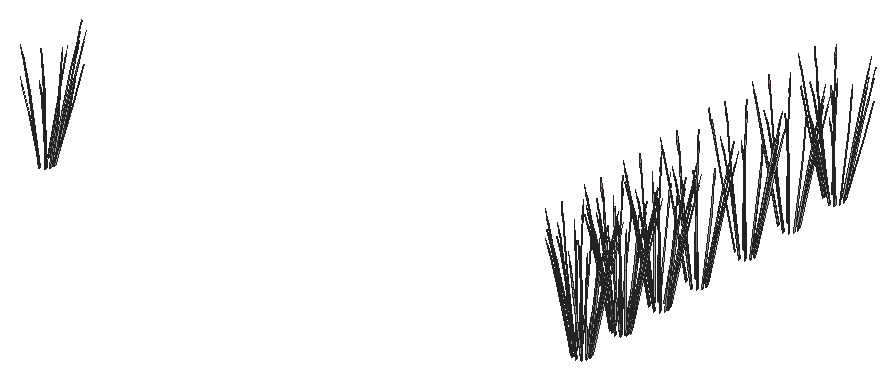
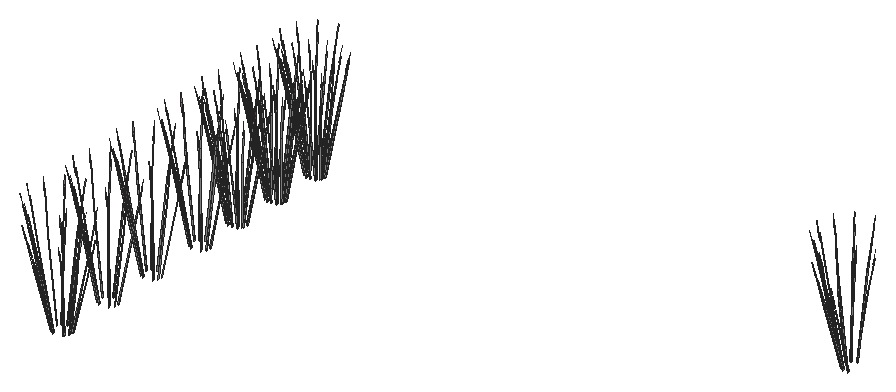
# SketchUp Ruby script. Lengths in inches.
U = 1.inch
M = Sketchup.active_model
def pt(a) = Geom::Point3d.new(a.map { |v| v * U })
def face(e, loops, mat)
  f = e.add_face(loops[0].map { |a| pt(a) })
  loops[1..].each { |l| e.add_face(l.map { |a| pt(a) }).erase! }
  f.material = f.back_material = mat if mat
  f
end
# faces: each face lists its corners as indices into pts; further lists are holes
def faces(e, pts, list, mat = nil) = list.each { |f| face(e, (f[0].is_a?(Array) ? f : [f]).map { |l| l.map { |i| pts[i] } }, mat) }
# xy, xz, yz: faces in a plane at the given z, y or x. An outline is a flat list of corners, or four numbers for a rectangle; further outlines are holes
def ring(l) = l.size == 4 ? [[l[0], l[1]], [l[2], l[1]], [l[2], l[3]], [l[0], l[3]]] : l.each_slice(2).to_a
def flat(e, list, mat, &to3) = list.each { |f| face(e, (f[0].is_a?(Array) ? f : [f]).map { |l| ring(l).map { |u, v| to3.(u, v) } }, mat) }
def xy(e, z, list, mat = nil) = flat(e, list, mat) { |x, y| [x, y, z] }
def xz(e, y, list, mat = nil) = flat(e, list, mat) { |x, z| [x, y, z] }
def yz(e, x, list, mat = nil) = flat(e, list, mat) { |y, z| [x, y, z] }
def lines(e, pts, list) = list.each { |a, b| e.add_line(pt(pts[a]), pt(pts[b])) }
# prism: a flat outline (further loops are holes) pulled along v
def prism(e, loops, v, mat = nil)
  f = face(e, loops, mat); d = Geom::Vector3d.new(v.map { |x| x * U })
  f.pushpull(f.normal.samedirection?(d) ? d.length : -d.length)
end
def box(e, o, s, mat = nil) = prism(e, [[o, [o[0] + s[0], o[1], o[2]], [o[0] + s[0], o[1] + s[1], o[2]], [o[0], o[1] + s[1], o[2]]]], [0, 0, s[2]], mat)
def at(x, y, z, deg = 0) = Geom::Transformation.translation(pt([x, y, z])) * Geom::Transformation.rotation(ORIGIN, Z_AXIS, deg.degrees)
def axes(o, x, y, z) = Geom::Transformation.new([*x, 0, *y, 0, *z, 0, *pt(o).to_a, 1])
def part(name) = M.definitions.add(name)
# library, detail: a bought-in or finely detailed component or shape, given as its bounding box
def library(name, o, s) = part(name).tap { |d| box(d.entities, o, s) }
def detail(e, o, s) = box(e.add_group.entities, o, s)
def put(e, d, t, mat = nil) = e.add_instance(d, t).tap { |i| i.material = mat if mat }
def group(e, t, mat = nil) = e.add_group.tap { |g| g.transformation = t; g.material = mat if mat }.entities
root = M.entities
M.materials.add("LightPink_Translucent").color = [144, 107, 117]
M.materials["LightPink_Translucent"].alpha = 0.75
M.materials.add("[_0053_Ivory_]").color = [200, 200, 200]
c1 = part("blade")
p = [[2.15,0.21,22],[0,0.17,0],[0.09,0.45,0],[2.18,0.31,22],[2.29,0.31,22],[0.38,0.45,0],
  [2.48,0.24,33],[2.49,0.24,33],[2.48,0.22,33]]
faces(c1.entities,p,[[0,1,2,3],[4,5,2,3],[6,3,4,7],[8,0,3,6]])
c2 = part("seeds")
p = [[0.3,-0.1,1.38],[-0.01,-0.03,1.59],[-0.01,-0.03,0.03],[0.14,-0.07,-0.07],[0.29,-0.03,3],[0.15,0.01,3.11]]
faces(c2.entities,p,[[0,1,2,3],[1,0,4,5]],"LightPink_Translucent")
c3 = part("blade with seeds")
put(c3.entities,c1,at(0,0,0))
put(c3.entities,c2,axes([2.4,0.25,30.99],[1.5799,-0.05474,1.17369],[-0.12525,1.92788,0.29478],[-0.07173,-0.02425,1.56792]))
put(root,c3,axes([483.9375,105.12,131.38],[-0.44753,0.21372,0.0643],[-0.21905,-0.38973,0.50621],[0.04322,0.1718,0.77189]),"[_0053_Ivory_]")
put(root,c3,axes([485.24,99.58,131.38],[0.44753,-0.21372,0.0643],[0.21905,0.38973,0.50621],[-0.04322,-0.1718,0.77189]),"[_0053_Ivory_]")
put(root,c3,axes([485.08,99.62,131.39],[0.59846,0.1644,0.48003],[-0.20464,0.54049,0.3958],[-0.03596,-0.21255,0.9933]),"[_0053_Ivory_]")
put(root,c3,axes([485.59,104.95,131.39],[-0.60408,0.14432,0.48003],[-0.10484,-0.56611,0.3958],[0.14207,0.16684,0.9933]),"[_0053_Ivory_]")
put(root,c3,axes([485.47,105.06,131.38],[-0.27604,0.39948,0.0643],[-0.39309,-0.23258,0.50621],[0.12709,0.12808,0.77189]),"[_0053_Ivory_]")
put(root,c3,axes([486.6,100.26,131.38],[0.49911,0.0293,0.0643],[-0.01368,0.44245,0.50621],[0.05223,-0.16948,0.77189]),"[_0053_Ivory_]")
put(root,c3,axes([486.44,100.22,131.39],[0.43249,0.42907,0.48003],[-0.45929,0.37004,0.3958],[0.07978,-0.2013,0.9933]),"[_0053_Ivory_]")
put(root,c3,axes([486.77,104.27,131.38],[-0.03058,0.47819,0.0643],[-0.4618,-0.01311,0.50621],[0.1769,0.05004,0.77189]),"[_0053_Ivory_]")
put(root,c3,axes([486.8125,104.12,131.39],[-0.44783,0.41436,0.48003],[-0.38623,-0.44004,0.3958],[0.21011,0.07643,0.9933]),"[_0053_Ivory_]")
put(root,c3,axes([487.42,101.5,131.38],[0.41695,0.26447,0.0643],[-0.24275,0.37662,0.50621],[0.13368,-0.12176,0.77189]),"[_0053_Ivory_]")
put(root,c3,axes([487.3,101.39,131.39],[0.15063,0.57876,0.48003],[-0.59087,0.10045,0.3958],[0.17414,-0.13612,0.9933]),"[_0053_Ivory_]")
put(root,c3,axes([487.48,102.97,131.38],[0.22307,0.42878,0.0643],[-0.40677,0.20987,0.50621],[0.17931,-0.04141,0.77189]),"[_0053_Ivory_]")
put(root,c3,axes([487.4375,102.82,131.39],[-0.17159,0.57338,0.48003],[-0.56413,-0.19607,0.3958],[0.22185,-0.03446,0.9933]),"[_0053_Ivory_]")
put(root,c3,axes([640.98,108.99,131.39],[0.17159,-0.57338,0.48003],[0.56413,0.19607,0.3958],[-0.22185,0.03446,0.9933]),"[_0053_Ivory_]")
put(root,c3,axes([640.98,124.05,131.39],[0.17159,-0.57338,0.48003],[0.56413,0.19607,0.3958],[-0.22185,0.03446,0.9933]),"[_0053_Ivory_]")
put(root,c3,axes([640.98,138.97,131.39],[0.17159,-0.57338,0.48003],[0.56413,0.19607,0.3958],[-0.22185,0.03446,0.9933]),"[_0053_Ivory_]")
put(root,c3,axes([640.98,153.24,131.39],[0.17159,-0.57338,0.48003],[0.56413,0.19607,0.3958],[-0.22185,0.03446,0.9933]),"[_0053_Ivory_]")
put(root,c3,axes([640.98,171.73,131.39],[0.17159,-0.57338,0.48003],[0.56413,0.19607,0.3958],[-0.22185,0.03446,0.9933]),"[_0053_Ivory_]")
put(root,c3,axes([640.98,188.49,131.39],[0.17159,-0.57338,0.48003],[0.56413,0.19607,0.3958],[-0.22185,0.03446,0.9933]),"[_0053_Ivory_]")
put(root,c3,axes([640.98,206.08,131.39],[0.17159,-0.57338,0.48003],[0.56413,0.19607,0.3958],[-0.22185,0.03446,0.9933]),"[_0053_Ivory_]")
put(root,c3,axes([640.93,205.93,131.38],[-0.22307,-0.42878,0.0643],[0.40677,-0.20987,0.50621],[-0.17931,0.04141,0.77189]),"[_0053_Ivory_]")
put(root,c3,axes([641.11,110.42,131.39],[-0.15063,-0.57876,0.48003],[0.59087,-0.10045,0.3958],[-0.17414,0.13612,0.9933]),"[_0053_Ivory_]")
put(root,c3,axes([641.11,125.48,131.39],[-0.15063,-0.57876,0.48003],[0.59087,-0.10045,0.3958],[-0.17414,0.13612,0.9933]),"[_0053_Ivory_]")
put(root,c3,axes([641.11,140.4,131.39],[-0.15063,-0.57876,0.48003],[0.59087,-0.10045,0.3958],[-0.17414,0.13612,0.9933]),"[_0053_Ivory_]")
put(root,c3,axes([641.11,154.67,131.39],[-0.15063,-0.57876,0.48003],[0.59087,-0.10045,0.3958],[-0.17414,0.13612,0.9933]),"[_0053_Ivory_]")
put(root,c3,axes([641.11,173.15,131.39],[-0.15063,-0.57876,0.48003],[0.59087,-0.10045,0.3958],[-0.17414,0.13612,0.9933]),"[_0053_Ivory_]")
put(root,c3,axes([641.11,189.91,131.39],[-0.15063,-0.57876,0.48003],[0.59087,-0.10045,0.3958],[-0.17414,0.13612,0.9933]),"[_0053_Ivory_]")
put(root,c3,axes([641.11,207.51,131.39],[-0.15063,-0.57876,0.48003],[0.59087,-0.10045,0.3958],[-0.17414,0.13612,0.9933]),"[_0053_Ivory_]")
put(root,c3,axes([641,207.39,131.38],[-0.41695,-0.26447,0.0643],[0.24275,-0.37662,0.50621],[-0.13368,0.12176,0.77189]),"[_0053_Ivory_]")
put(root,c3,axes([641.39,108.99,131.7],[0.50475,0.17543,0.35414],[-0.14722,0.5118,-0.4572],[-0.20322,0.04693,0.87481]),"[_0053_Ivory_]")
put(root,c3,axes([641.39,124.06,131.7],[0.50475,0.17543,0.35414],[-0.14722,0.5118,-0.4572],[-0.20322,0.04693,0.87481]),"[_0053_Ivory_]")
put(root,c3,axes([641.96,107.89,131.7],[0.34557,0.39372,0.35414],[-0.39459,0.37271,-0.4572],[-0.20048,-0.05671,0.87481]),"[_0053_Ivory_]")
put(root,c3,axes([641.96,122.95,131.7],[0.34557,0.39372,0.35414],[-0.39459,0.37271,-0.4572],[-0.20048,-0.05671,0.87481]),"[_0053_Ivory_]")
put(root,c3,axes([641.96,137.87,131.7],[0.34557,0.39372,0.35414],[-0.39459,0.37271,-0.4572],[-0.20048,-0.05671,0.87481]),"[_0053_Ivory_]")
put(root,c3,axes([641.48,110.22,131.7],[0.52868,-0.08987,0.35414],[0.1396,0.51376,-0.4572],[-0.1515,0.13799,0.87481]),"[_0053_Ivory_]")
put(root,c3,axes([641.48,125.29,131.7],[0.52868,-0.08987,0.35414],[0.1396,0.51376,-0.4572],[-0.1515,0.13799,0.87481]),"[_0053_Ivory_]")
put(root,c3,axes([641.48,140.2,131.7],[0.52868,-0.08987,0.35414],[0.1396,0.51376,-0.4572],[-0.1515,0.13799,0.87481]),"[_0053_Ivory_]")
put(root,c3,axes([641.98,111.59,131.39],[-0.43249,-0.42907,0.48003],[0.45929,-0.37004,0.3958],[-0.07978,0.2013,0.9933]),"[_0053_Ivory_]")
put(root,c3,axes([641.98,126.65,131.39],[-0.43249,-0.42907,0.48003],[0.45929,-0.37004,0.3958],[-0.07978,0.2013,0.9933]),"[_0053_Ivory_]")
put(root,c3,axes([641.98,141.57,131.39],[-0.43249,-0.42907,0.48003],[0.45929,-0.37004,0.3958],[-0.07978,0.2013,0.9933]),"[_0053_Ivory_]")
put(root,c3,axes([641.98,155.84,131.39],[-0.43249,-0.42907,0.48003],[0.45929,-0.37004,0.3958],[-0.07978,0.2013,0.9933]),"[_0053_Ivory_]")
put(root,c3,axes([641.98,174.33,131.39],[-0.43249,-0.42907,0.48003],[0.45929,-0.37004,0.3958],[-0.07978,0.2013,0.9933]),"[_0053_Ivory_]")
put(root,c3,axes([641.98,191.09,131.39],[-0.43249,-0.42907,0.48003],[0.45929,-0.37004,0.3958],[-0.07978,0.2013,0.9933]),"[_0053_Ivory_]")
put(root,c3,axes([641.98,208.68,131.39],[-0.43249,-0.42907,0.48003],[0.45929,-0.37004,0.3958],[-0.07978,0.2013,0.9933]),"[_0053_Ivory_]")
put(root,c3,axes([641.82,208.64,131.38],[-0.49911,-0.0293,0.0643],[0.01368,-0.44245,0.50621],[-0.05223,0.16948,0.77189]),"[_0053_Ivory_]")
put(root,c3,axes([643.03,107.21,131.7],[0.0938,0.50652,0.35414],[-0.53623,0.13375,-0.4572],[-0.14403,-0.14515,0.87481]),"[_0053_Ivory_]")
put(root,c3,axes([643.03,122.27,131.7],[0.0938,0.50652,0.35414],[-0.53623,0.13375,-0.4572],[-0.14403,-0.14515,0.87481]),"[_0053_Ivory_]")
put(root,c3,axes([642.1875,111.25,131.7],[0.41095,-0.33109,0.35414],[0.38901,0.37805,-0.4572],[-0.05919,0.19208,0.87481]),"[_0053_Ivory_]")
put(root,c3,axes([642.1875,126.3125,131.7],[0.41095,-0.33109,0.35414],[0.38901,0.37805,-0.4572],[-0.05919,0.19208,0.87481]),"[_0053_Ivory_]")
put(root,c3,axes([642.1875,141.23,131.7],[0.41095,-0.33109,0.35414],[0.38901,0.37805,-0.4572],[-0.05919,0.19208,0.87481]),"[_0053_Ivory_]")
put(root,c3,axes([644.31,107.125,131.7],[-0.1831,0.48359,0.35414],[-0.53419,-0.14105,-0.4572],[-0.04898,-0.1947,0.87481]),"[_0053_Ivory_]")
put(root,c3,axes([644.31,122.19,131.7],[-0.1831,0.48359,0.35414],[-0.53419,-0.14105,-0.4572],[-0.04898,-0.1947,0.87481]),"[_0053_Ivory_]")
put(root,c3,axes([644.31,137.11,131.7],[-0.1831,0.48359,0.35414],[-0.53419,-0.14105,-0.4572],[-0.04898,-0.1947,0.87481]),"[_0053_Ivory_]")
put(root,c3,axes([644.48,203.78,131.38],[0.44753,-0.21372,0.0643],[0.21905,0.38973,0.50621],[-0.04322,-0.1718,0.77189]),"[_0053_Ivory_]")
put(root,c3,axes([644.32,106.73,131.39],[0.59846,0.1644,0.48003],[-0.20464,0.54049,0.3958],[-0.03596,-0.21255,0.9933]),"[_0053_Ivory_]")
put(root,c3,axes([644.32,121.79,131.39],[0.59846,0.1644,0.48003],[-0.20464,0.54049,0.3958],[-0.03596,-0.21255,0.9933]),"[_0053_Ivory_]")
put(root,c3,axes([644.32,136.71,131.39],[0.59846,0.1644,0.48003],[-0.20464,0.54049,0.3958],[-0.03596,-0.21255,0.9933]),"[_0053_Ivory_]")
put(root,c3,axes([644.32,150.98,131.39],[0.59846,0.1644,0.48003],[-0.20464,0.54049,0.3958],[-0.03596,-0.21255,0.9933]),"[_0053_Ivory_]")
put(root,c3,axes([644.32,169.47,131.39],[0.59846,0.1644,0.48003],[-0.20464,0.54049,0.3958],[-0.03596,-0.21255,0.9933]),"[_0053_Ivory_]")
put(root,c3,axes([644.32,186.23,131.39],[0.59846,0.1644,0.48003],[-0.20464,0.54049,0.3958],[-0.03596,-0.21255,0.9933]),"[_0053_Ivory_]")
put(root,c3,axes([644.32,203.82,131.39],[0.59846,0.1644,0.48003],[-0.20464,0.54049,0.3958],[-0.03596,-0.21255,0.9933]),"[_0053_Ivory_]")
put(root,c3,axes([643.34,111.79,131.7],[0.1831,-0.48359,0.35414],[0.53419,0.14105,-0.4572],[0.04898,0.1947,0.87481]),"[_0053_Ivory_]")
put(root,c3,axes([643.34,126.86,131.7],[0.1831,-0.48359,0.35414],[0.53419,0.14105,-0.4572],[0.04898,0.1947,0.87481]),"[_0053_Ivory_]")
put(root,c3,axes([643.34,141.77,131.7],[0.1831,-0.48359,0.35414],[0.53419,0.14105,-0.4572],[0.04898,0.1947,0.87481]),"[_0053_Ivory_]")
put(root,c3,axes([645.46,107.67,131.7],[-0.41095,0.33109,0.35414],[-0.38901,-0.37805,-0.4572],[0.05919,-0.19208,0.87481]),"[_0053_Ivory_]")
put(root,c3,axes([645.46,122.73,131.7],[-0.41095,0.33109,0.35414],[-0.38901,-0.37805,-0.4572],[0.05919,-0.19208,0.87481]),"[_0053_Ivory_]")
put(root,c3,axes([644.82,112.06,131.39],[-0.60408,0.14432,0.48003],[-0.10484,-0.56611,0.3958],[0.14207,0.16684,0.9933]),"[_0053_Ivory_]")
put(root,c3,axes([644.82,127.12,131.39],[-0.60408,0.14432,0.48003],[-0.10484,-0.56611,0.3958],[0.14207,0.16684,0.9933]),"[_0053_Ivory_]")
put(root,c3,axes([644.82,142.04,131.39],[-0.60408,0.14432,0.48003],[-0.10484,-0.56611,0.3958],[0.14207,0.16684,0.9933]),"[_0053_Ivory_]")
put(root,c3,axes([644.82,156.3125,131.39],[-0.60408,0.14432,0.48003],[-0.10484,-0.56611,0.3958],[0.14207,0.16684,0.9933]),"[_0053_Ivory_]")
put(root,c3,axes([644.82,174.8,131.39],[-0.60408,0.14432,0.48003],[-0.10484,-0.56611,0.3958],[0.14207,0.16684,0.9933]),"[_0053_Ivory_]")
put(root,c3,axes([644.82,191.56,131.39],[-0.60408,0.14432,0.48003],[-0.10484,-0.56611,0.3958],[0.14207,0.16684,0.9933]),"[_0053_Ivory_]")
put(root,c3,axes([644.82,209.15,131.39],[-0.60408,0.14432,0.48003],[-0.10484,-0.56611,0.3958],[0.14207,0.16684,0.9933]),"[_0053_Ivory_]")
put(root,c3,axes([644.71,209.26,131.38],[-0.27604,0.39948,0.0643],[-0.39309,-0.23258,0.50621],[0.12709,0.12808,0.77189]),"[_0053_Ivory_]")
put(root,c3,axes([644.625,111.71,131.7],[-0.0938,-0.50652,0.35414],[0.53623,-0.13375,-0.4572],[0.14403,0.14515,0.87481]),"[_0053_Ivory_]")
put(root,c3,axes([644.625,126.77,131.7],[-0.0938,-0.50652,0.35414],[0.53623,-0.13375,-0.4572],[0.14403,0.14515,0.87481]),"[_0053_Ivory_]")
put(root,c3,axes([645.84,204.46,131.38],[0.49911,0.0293,0.0643],[-0.01368,0.44245,0.50621],[0.05223,-0.16948,0.77189]),"[_0053_Ivory_]")
put(root,c3,axes([645.68,107.33,131.39],[0.43249,0.42907,0.48003],[-0.45929,0.37004,0.3958],[0.07978,-0.2013,0.9933]),"[_0053_Ivory_]")
put(root,c3,axes([645.68,122.39,131.39],[0.43249,0.42907,0.48003],[-0.45929,0.37004,0.3958],[0.07978,-0.2013,0.9933]),"[_0053_Ivory_]")
put(root,c3,axes([645.68,137.31,131.39],[0.43249,0.42907,0.48003],[-0.45929,0.37004,0.3958],[0.07978,-0.2013,0.9933]),"[_0053_Ivory_]")
put(root,c3,axes([645.68,151.59,131.39],[0.43249,0.42907,0.48003],[-0.45929,0.37004,0.3958],[0.07978,-0.2013,0.9933]),"[_0053_Ivory_]")
put(root,c3,axes([645.68,170.07,131.39],[0.43249,0.42907,0.48003],[-0.45929,0.37004,0.3958],[0.07978,-0.2013,0.9933]),"[_0053_Ivory_]")
put(root,c3,axes([645.68,186.83,131.39],[0.43249,0.42907,0.48003],[-0.45929,0.37004,0.3958],[0.07978,-0.2013,0.9933]),"[_0053_Ivory_]")
put(root,c3,axes([645.68,204.42,131.39],[0.43249,0.42907,0.48003],[-0.45929,0.37004,0.3958],[0.07978,-0.2013,0.9933]),"[_0053_Ivory_]")
put(root,c3,axes([646.18,108.69,131.7],[-0.52868,0.08987,0.35414],[-0.1396,-0.51376,-0.4572],[0.1515,-0.13799,0.87481]),"[_0053_Ivory_]")
put(root,c3,axes([646.18,123.76,131.7],[-0.52868,0.08987,0.35414],[-0.1396,-0.51376,-0.4572],[0.1515,-0.13799,0.87481]),"[_0053_Ivory_]")
put(root,c3,axes([645.69,111.03,131.7],[-0.34557,-0.39372,0.35414],[0.39459,-0.37271,-0.4572],[0.20048,0.05671,0.87481]),"[_0053_Ivory_]")
put(root,c3,axes([645.69,126.09,131.7],[-0.34557,-0.39372,0.35414],[0.39459,-0.37271,-0.4572],[0.20048,0.05671,0.87481]),"[_0053_Ivory_]")
put(root,c3,axes([645.69,141.01,131.7],[-0.34557,-0.39372,0.35414],[0.39459,-0.37271,-0.4572],[0.20048,0.05671,0.87481]),"[_0053_Ivory_]")
put(root,c3,axes([646.01,208.47,131.38],[-0.03058,0.47819,0.0643],[-0.4618,-0.01311,0.50621],[0.1769,0.05004,0.77189]),"[_0053_Ivory_]")
put(root,c3,axes([646.05,111.23,131.39],[-0.44783,0.41436,0.48003],[-0.38623,-0.44004,0.3958],[0.21011,0.07643,0.9933]),"[_0053_Ivory_]")
put(root,c3,axes([646.05,126.3,131.39],[-0.44783,0.41436,0.48003],[-0.38623,-0.44004,0.3958],[0.21011,0.07643,0.9933]),"[_0053_Ivory_]")
put(root,c3,axes([646.05,141.21,131.39],[-0.44783,0.41436,0.48003],[-0.38623,-0.44004,0.3958],[0.21011,0.07643,0.9933]),"[_0053_Ivory_]")
put(root,c3,axes([646.05,155.49,131.39],[-0.44783,0.41436,0.48003],[-0.38623,-0.44004,0.3958],[0.21011,0.07643,0.9933]),"[_0053_Ivory_]")
put(root,c3,axes([646.05,173.97,131.39],[-0.44783,0.41436,0.48003],[-0.38623,-0.44004,0.3958],[0.21011,0.07643,0.9933]),"[_0053_Ivory_]")
put(root,c3,axes([646.05,190.73,131.39],[-0.44783,0.41436,0.48003],[-0.38623,-0.44004,0.3958],[0.21011,0.07643,0.9933]),"[_0053_Ivory_]")
put(root,c3,axes([646.05,208.32,131.39],[-0.44783,0.41436,0.48003],[-0.38623,-0.44004,0.3958],[0.21011,0.07643,0.9933]),"[_0053_Ivory_]")
put(root,c3,axes([646.26,109.92,131.7],[-0.50475,-0.17543,0.35414],[0.14722,-0.5118,-0.4572],[0.20322,-0.04693,0.87481]),"[_0053_Ivory_]")
put(root,c3,axes([646.26,124.99,131.7],[-0.50475,-0.17543,0.35414],[0.14722,-0.5118,-0.4572],[0.20322,-0.04693,0.87481]),"[_0053_Ivory_]")
put(root,c3,axes([646.26,139.9,131.7],[-0.50475,-0.17543,0.35414],[0.14722,-0.5118,-0.4572],[0.20322,-0.04693,0.87481]),"[_0053_Ivory_]")
put(root,c3,axes([646.54,108.5,131.39],[0.15063,0.57876,0.48003],[-0.59087,0.10045,0.3958],[0.17414,-0.13612,0.9933]),"[_0053_Ivory_]")
put(root,c3,axes([646.54,123.57,131.39],[0.15063,0.57876,0.48003],[-0.59087,0.10045,0.3958],[0.17414,-0.13612,0.9933]),"[_0053_Ivory_]")
put(root,c3,axes([646.54,138.48,131.39],[0.15063,0.57876,0.48003],[-0.59087,0.10045,0.3958],[0.17414,-0.13612,0.9933]),"[_0053_Ivory_]")
put(root,c3,axes([646.54,152.76,131.39],[0.15063,0.57876,0.48003],[-0.59087,0.10045,0.3958],[0.17414,-0.13612,0.9933]),"[_0053_Ivory_]")
put(root,c3,axes([646.54,171.24,131.39],[0.15063,0.57876,0.48003],[-0.59087,0.10045,0.3958],[0.17414,-0.13612,0.9933]),"[_0053_Ivory_]")
put(root,c3,axes([646.54,188,131.39],[0.15063,0.57876,0.48003],[-0.59087,0.10045,0.3958],[0.17414,-0.13612,0.9933]),"[_0053_Ivory_]")
put(root,c3,axes([646.54,205.59,131.39],[0.15063,0.57876,0.48003],[-0.59087,0.10045,0.3958],[0.17414,-0.13612,0.9933]),"[_0053_Ivory_]")
put(root,c3,axes([646.68,109.93,131.39],[-0.17159,0.57338,0.48003],[-0.56413,-0.19607,0.3958],[0.22185,-0.03446,0.9933]),"[_0053_Ivory_]")
put(root,c3,axes([646.68,124.99,131.39],[-0.17159,0.57338,0.48003],[-0.56413,-0.19607,0.3958],[0.22185,-0.03446,0.9933]),"[_0053_Ivory_]")
put(root,c3,axes([646.68,139.91,131.39],[-0.17159,0.57338,0.48003],[-0.56413,-0.19607,0.3958],[0.22185,-0.03446,0.9933]),"[_0053_Ivory_]")
put(root,c3,axes([646.68,154.19,131.39],[-0.17159,0.57338,0.48003],[-0.56413,-0.19607,0.3958],[0.22185,-0.03446,0.9933]),"[_0053_Ivory_]")
put(root,c3,axes([646.68,172.67,131.39],[-0.17159,0.57338,0.48003],[-0.56413,-0.19607,0.3958],[0.22185,-0.03446,0.9933]),"[_0053_Ivory_]")
put(root,c3,axes([646.68,189.43,131.39],[-0.17159,0.57338,0.48003],[-0.56413,-0.19607,0.3958],[0.22185,-0.03446,0.9933]),"[_0053_Ivory_]")
put(root,c3,axes([646.68,207.02,131.39],[-0.17159,0.57338,0.48003],[-0.56413,-0.19607,0.3958],[0.22185,-0.03446,0.9933]),"[_0053_Ivory_]")
